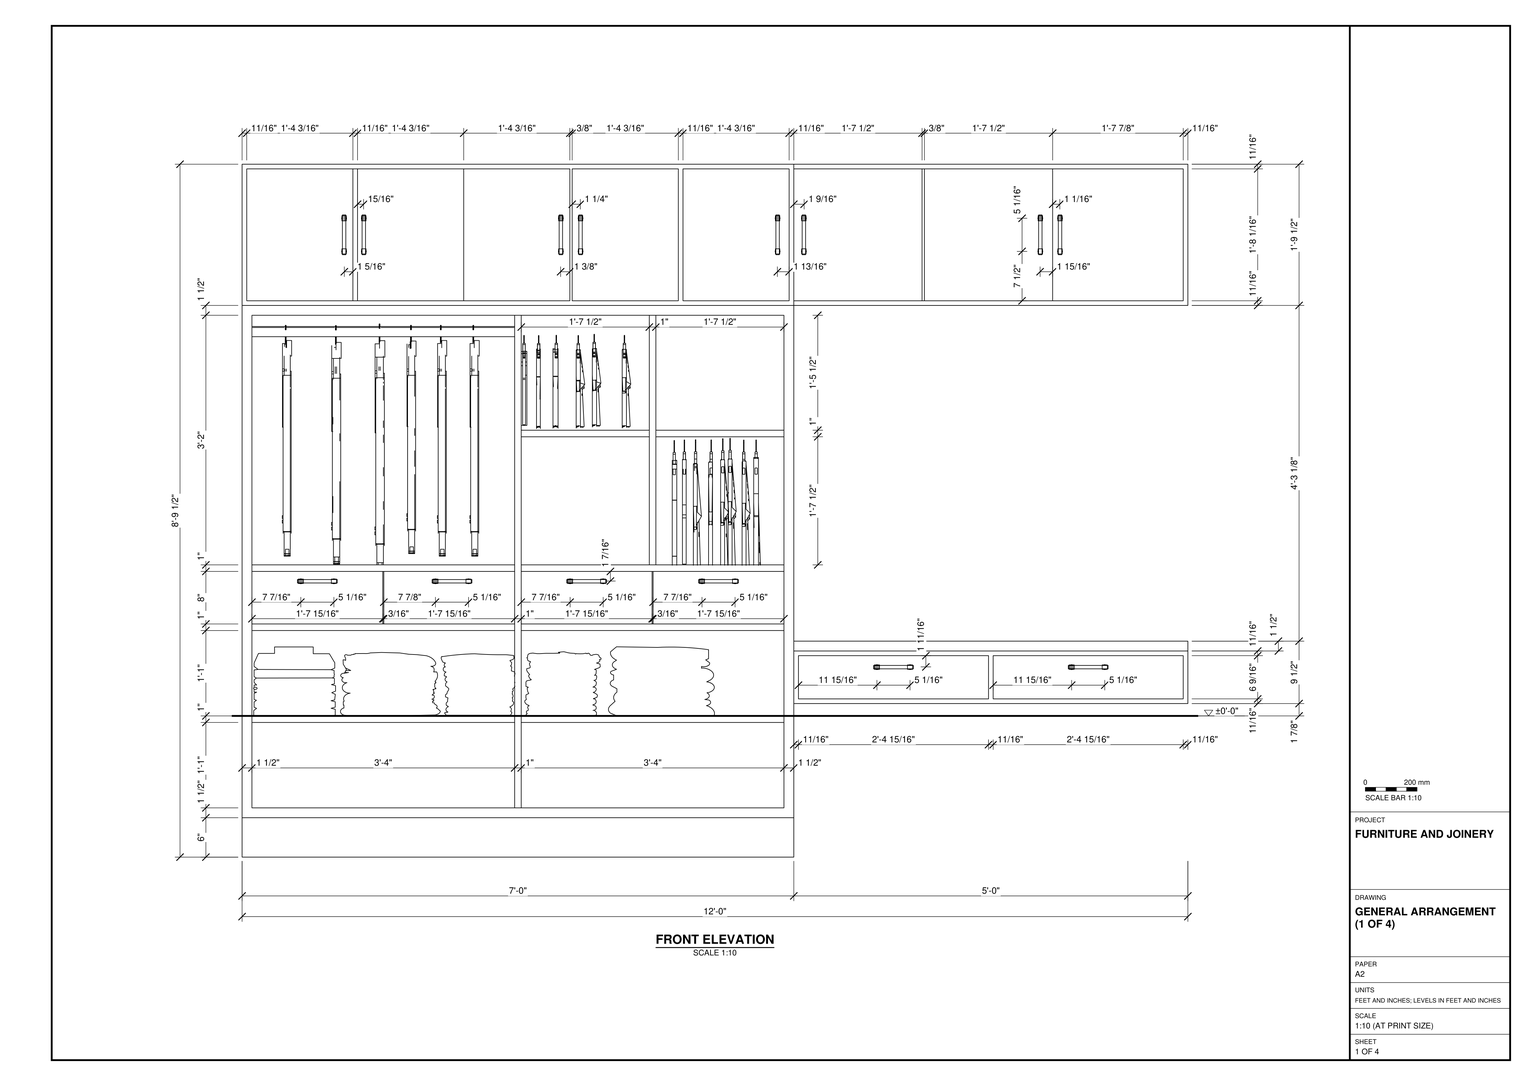
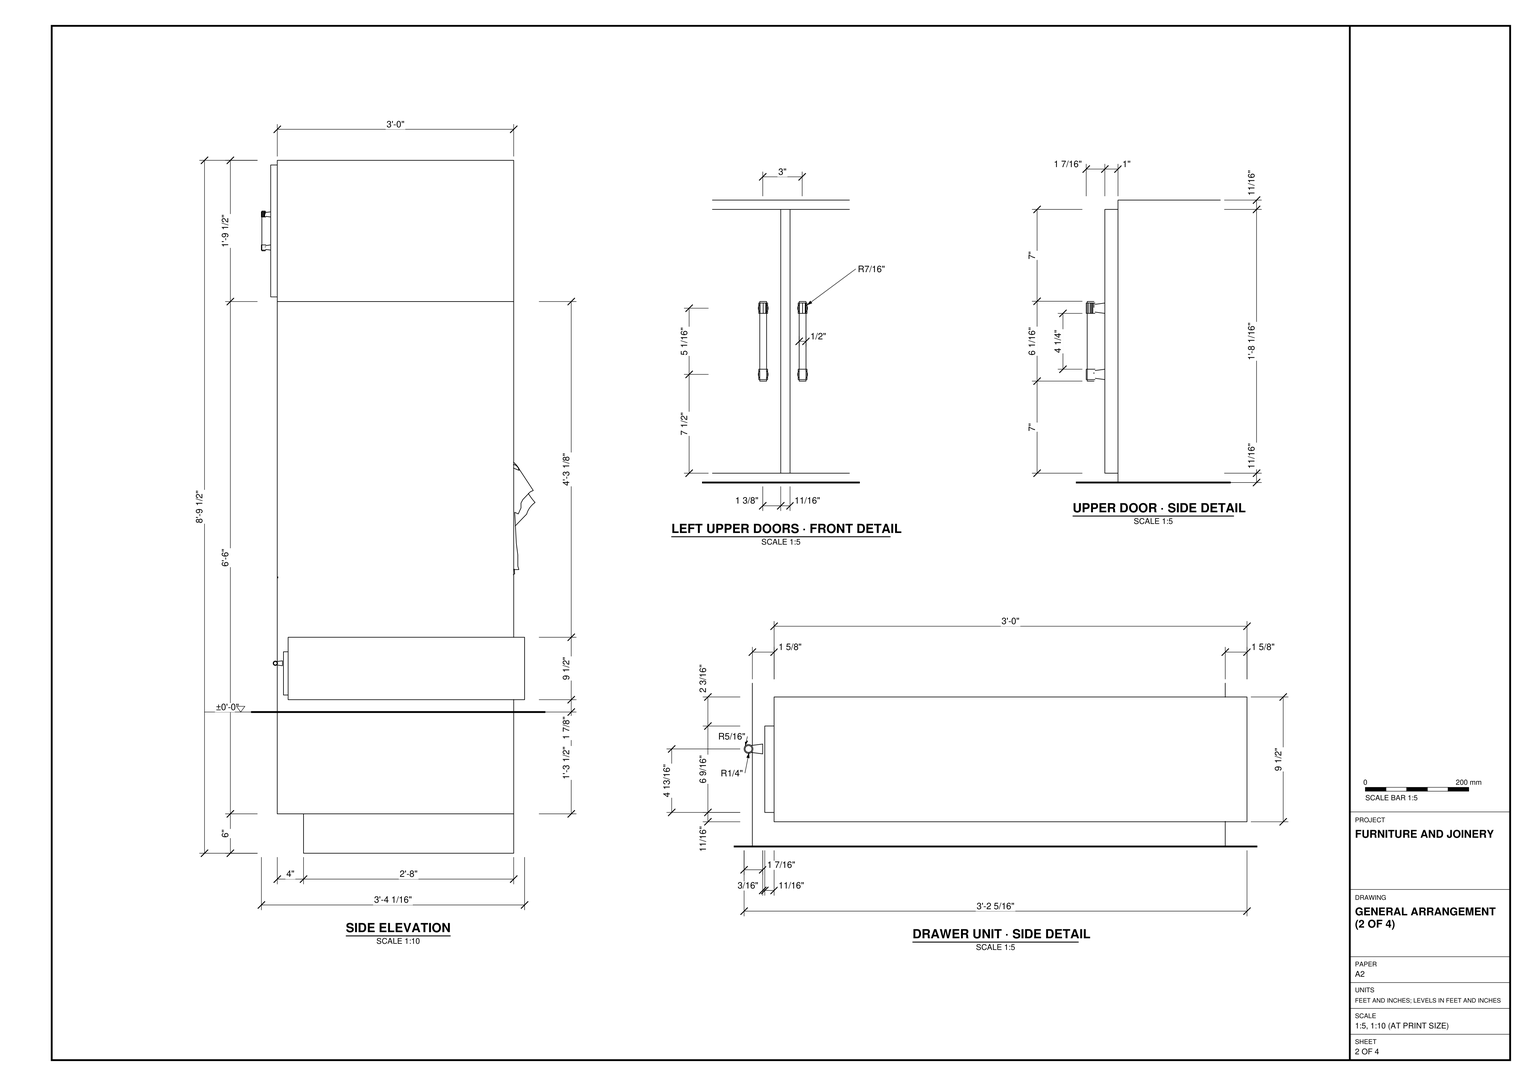
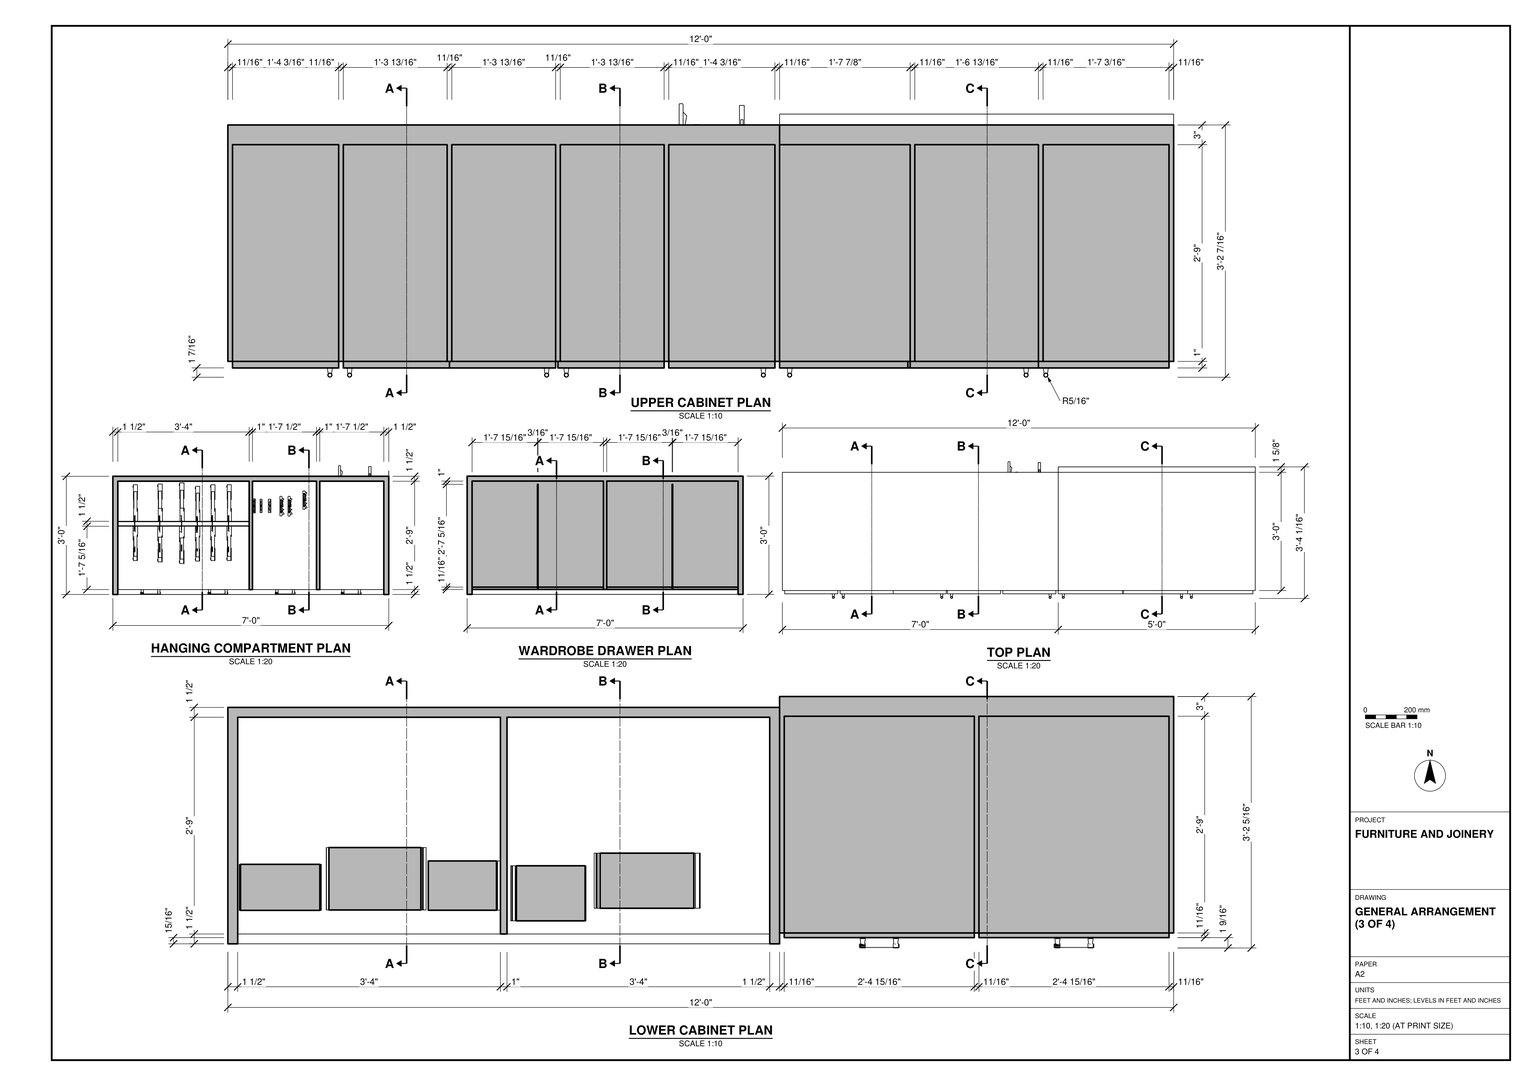
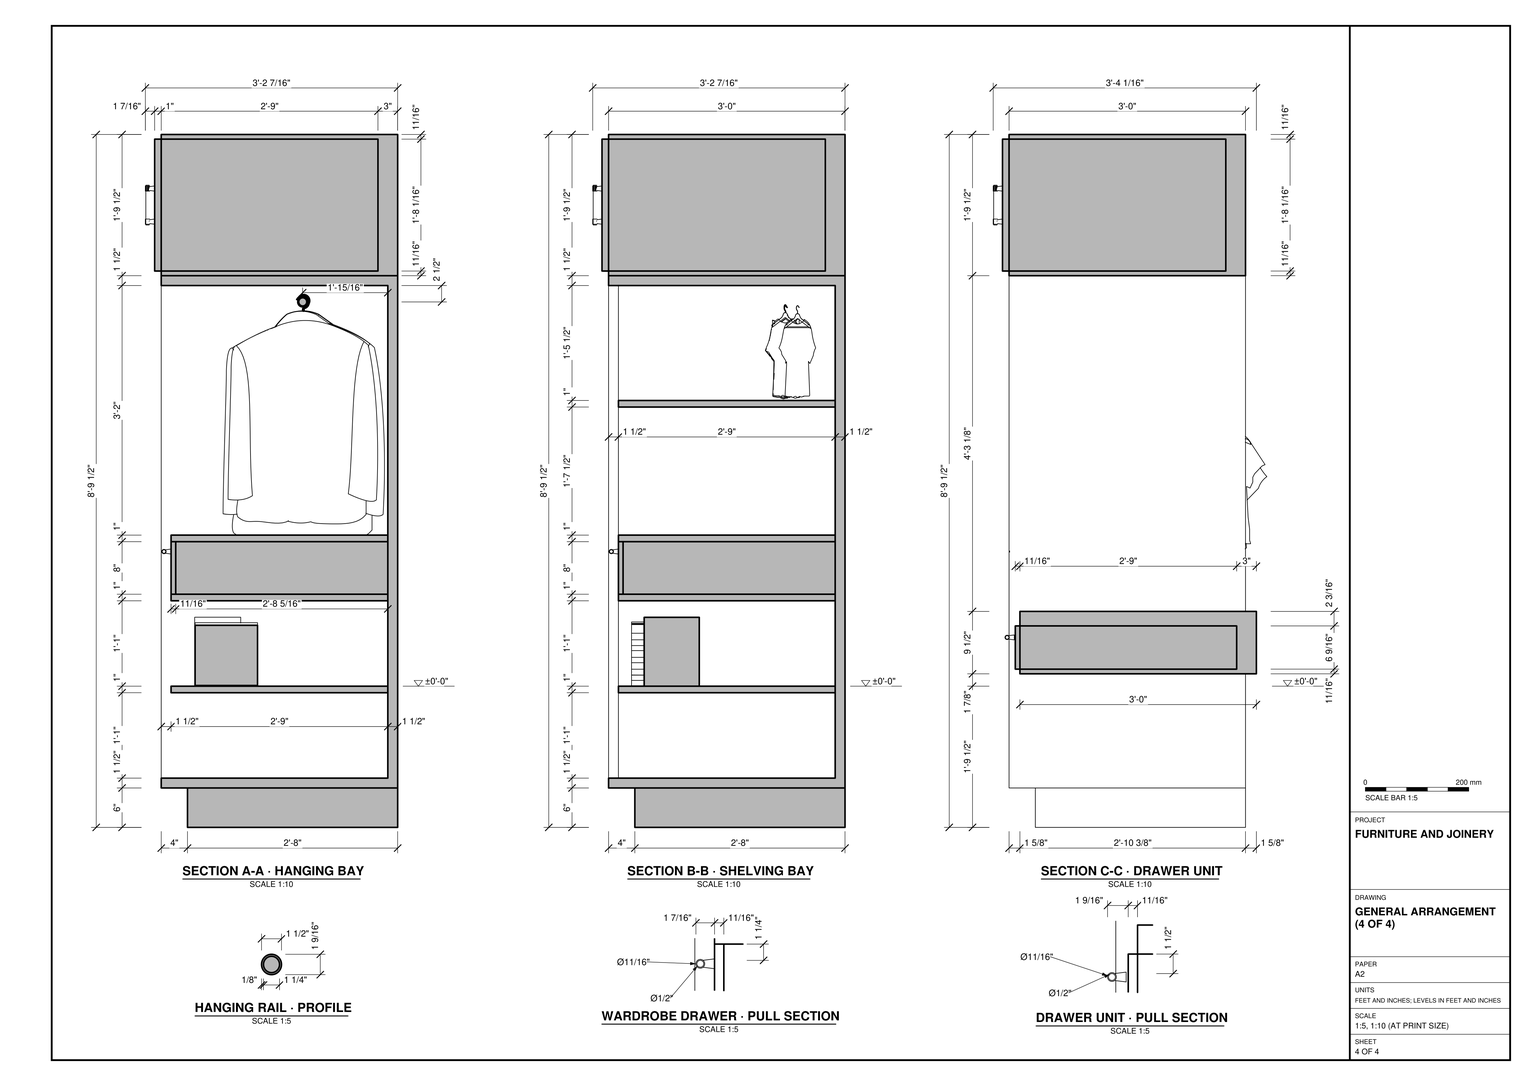
Build the wardrobe assembly in SketchUp from task_files/diagram_01.pdf. Work in feet and inches. The complete assembly is 12'-0" wide, 3'-5 11/16" deep and 8'-9 1/2" high. Use the ±0'-0" datum shown in the elevations; the wardrobe plinth sits below this line.

Set out the 7'-0" wardrobe on the left and the 5'-0" drawer unit on the right. Run the upper cabinets across both sections, following the door widths and pull positions in the front elevation. Below the left cabinets, form a wide bay for long garments and two narrower bays with intermediate shelves. Fit the row of drawers beneath the hanging bays, with divided open shelving and a recessed plinth below. On the right, leave the space between the suspended two-drawer unit and the overhead cabinets open. Use the plans and side details to set the panel thicknesses, front projections and pull orientations.

Place hanging garments and folded clothing in the compartments shown. Decor and loose items, including the clothing, may be any suitable library components. Keep each joinery piece in a separate group or component and use components for repeated parts such as matching pulls. Save one SketchUp model as output_files/wardrobe_with_overhead_cabinets_and_suspended_drawers.skp.

# SketchUp Ruby script. Lengths in inches.
U = 1.inch
M = Sketchup.active_model
def pt(a) = Geom::Point3d.new(a.map { |v| v * U })
def face(e, loops, mat)
  f = e.add_face(loops[0].map { |a| pt(a) })
  loops[1..].each { |l| e.add_face(l.map { |a| pt(a) }).erase! }
  f.material = f.back_material = mat if mat
  f
end
# faces: each face lists its corners as indices into pts; further lists are holes
def faces(e, pts, list, mat = nil) = list.each { |f| face(e, (f[0].is_a?(Array) ? f : [f]).map { |l| l.map { |i| pts[i] } }, mat) }
# xy, xz, yz: faces in a plane at the given z, y or x. An outline is a flat list of corners, or four numbers for a rectangle; further outlines are holes
def ring(l) = l.size == 4 ? [[l[0], l[1]], [l[2], l[1]], [l[2], l[3]], [l[0], l[3]]] : l.each_slice(2).to_a
def flat(e, list, mat, &to3) = list.each { |f| face(e, (f[0].is_a?(Array) ? f : [f]).map { |l| ring(l).map { |u, v| to3.(u, v) } }, mat) }
def xy(e, z, list, mat = nil) = flat(e, list, mat) { |x, y| [x, y, z] }
def xz(e, y, list, mat = nil) = flat(e, list, mat) { |x, z| [x, y, z] }
def yz(e, x, list, mat = nil) = flat(e, list, mat) { |y, z| [x, y, z] }
def lines(e, pts, list) = list.each { |a, b| e.add_line(pt(pts[a]), pt(pts[b])) }
# prism: a flat outline (further loops are holes) pulled along v
def prism(e, loops, v, mat = nil)
  f = face(e, loops, mat); d = Geom::Vector3d.new(v.map { |x| x * U })
  f.pushpull(f.normal.samedirection?(d) ? d.length : -d.length)
end
def box(e, o, s, mat = nil) = prism(e, [[o, [o[0] + s[0], o[1], o[2]], [o[0] + s[0], o[1] + s[1], o[2]], [o[0], o[1] + s[1], o[2]]]], [0, 0, s[2]], mat)
def at(x, y, z, deg = 0) = Geom::Transformation.translation(pt([x, y, z])) * Geom::Transformation.rotation(ORIGIN, Z_AXIS, deg.degrees)
def axes(o, x, y, z) = Geom::Transformation.new([*x, 0, *y, 0, *z, 0, *pt(o).to_a, 1])
def part(name) = M.definitions.add(name)
# library, detail: a bought-in or finely detailed component or shape, given as its bounding box
def library(name, o, s) = part(name).tap { |d| box(d.entities, o, s) }
def detail(e, o, s) = box(e.add_group.entities, o, s)
def put(e, d, t, mat = nil) = e.add_instance(d, t).tap { |i| i.material = mat if mat }
def group(e, t, mat = nil) = e.add_group.tap { |g| g.transformation = t; g.material = mat if mat }.entities
root = M.entities
c1 = library("1-POIGNEE CLC2",[-3.03,-0.375,0],[6.06,0.75,1.42])
c2 = library("clothing6",[65.37,-6.9,0.1],[26.12,44.83,39.07])
c3 = library("clothing (1)",[291.68,-309.73,41.26],[36.47,20.09,38.36])
c4 = library("Component",[186.95,333.1,21.5],[70.2,11.17,10.52])
c5 = part("Group\#3")
box(c5.entities,[0,0,0],[19.5,33,1])
c6 = part("Group\#7")
box(c6.entities,[0,0,0],[40,33,1])
c7 = part("Group\#14")
box(c7.entities,[0,0,0],[16.16,1,20.08])
c8 = part("Group\#13")
put(c8.entities,c7,at(0,-1,0))
c9 = part("Group\#16")
box(c9.entities,[0,-1,0],[19.88,1,20.08])
c10 = part("Group\#18")
box(c10.entities,[0,-0.71,0],[28.9375,0.71,6.58])
c11 = part("Group\#20")
box(c11.entities,[0,-0.71,0],[19.92,0.71,8])
prism(root,[[[1.5,35.5,35.5],[41.5,35.5,35.5],[41.5,3.21,35.5],[21.58,3.21,35.5],[21.58,34.5,35.5],[21.42,34.5,35.5],[21.42,3.21,35.5],[1.5,3.21,35.5]]],[0,0,8])
p = [[62,35.5,82.5],[62,35.5,44.5],[63,35.5,82.5],[63,35.5,44.5]]
lines(root,p,[[0,1],[2,3]])
put(root,c1,axes([11.46,2.5,42],[1,0,0],[0,0,1],[0,-1,0]))
put(root,c1,axes([31.96,2.5,42],[1,0,0],[0,0,1],[0,-1,0]))
put(root,c1,axes([52.46,2.5,42],[1,0,0],[0,0,1],[0,-1,0]))
put(root,c1,axes([72.54,2.5,42],[1,0,0],[0,0,1],[0,-1,0]))
put(root,c1,axes([99.18,1.79,28.93],[1,0,0],[0,0,1],[0,-1,0]))
put(root,c1,axes([15.53,0,94.75],[0,0,-1],[1,0,0],[0,-1,0]))
put(root,c1,axes([128.82,1.79,28.93],[1,0,0],[0,0,1],[0,-1,0]))
put(root,c1,axes([18.53,0,94.75],[0,0,-1],[1,0,0],[0,-1,0]))
put(root,c1,axes([48.53,0,94.75],[0,0,-1],[1,0,0],[0,-1,0]))
put(root,c1,axes([51.53,0,94.75],[0,0,-1],[1,0,0],[0,-1,0]))
put(root,c1,axes([81.53,0,94.75],[0,0,-1],[1,0,0],[0,-1,0]))
put(root,c1,axes([85.53,0,94.75],[0,0,-1],[1,0,0],[0,-1,0]))
put(root,c1,axes([121.53,0,94.75],[0,0,-1],[1,0,0],[0,-1,0]))
put(root,c1,axes([124.53,0,94.75],[0,0,-1],[1,0,0],[0,-1,0]))
put(root,c2,axes([7.66,96.49,43.61],[0,-0.9408,0],[0.89234,0,0],[0,0,0.95962]))
put(root,c3,at(-249.18,329.89,0))
put(root,c4,at(-185.22,-328.6,0))
put(root,c5,at(42.5,2.5,64))
g1 = group(root,at(42.5,2.5,43.5))
box(g1,[0,0,0],[40,33,1])
g2 = group(root,at(0,37,6))
xy(g2,0,[[0,-36,84,0]])
xy(g2,1.5,[[1.5,-36,82.5,-36,82.5,-1.5,42.5,-1.5,42.5,-34.5,41.5,-34.5,41.5,-1.5,1.5,-1.5]])
xy(g2,38.5,[[62,-34.5,63,-1.5]])
xy(g2,76.5,[[1.5,-36,1.5,-1.5,41.5,-1.5,41.5,-34.5,42.5,-34.5,42.5,-1.5,62,-1.5,62,-34.5,63,-34.5,63,-1.5,82.5,-1.5,82.5,-36]])
xy(g2,78,[[0,-36,84,0]])
xz(g2,-36,[[[0,0,84,78],[1.5,1.5,82.5,76.5]]])
xz(g2,-34.5,[[41.5,1.5,42.5,76.5],[62,38.5,63,76.5]])
xz(g2,-1.5,[[1.5,1.5,41.5,76.5],[42.5,1.5,82.5,1.5,82.5,76.5,63,76.5,63,38.5,62,38.5,62,76.5,42.5,76.5]])
xz(g2,0,[[0,0,84,78]])
yz(g2,0,[[-36,0,0,78]])
yz(g2,1.5,[[-36,1.5,-1.5,76.5]])
yz(g2,41.5,[[-34.5,1.5,-1.5,76.5]])
yz(g2,42.5,[[-34.5,1.5,-1.5,76.5]])
yz(g2,62,[[-34.5,38.5,-1.5,76.5]])
yz(g2,63,[[-34.5,38.5,-1.5,76.5]])
yz(g2,82.5,[[-36,1.5,-1.5,76.5]])
yz(g2,84,[[-36,0,0,78]])
put(root,c6,at(42.5,2.5,20.5))
g3 = group(root,at(42.5,2.5,34.5))
box(g3,[0,0,0],[40,33,1])
put(root,c6,at(1.5,2.5,20.5))
put(root,c6,at(1.5,2.5,34.5))
g4 = group(root,at(0,1,0))
box(g4,[0,4,0],[84,32,6])
put(root,c5,at(63,2.5,64))
g5 = group(root,at(42.5,35.5,35.5))
xy(g5,0,[[0,-32.29,0,0,40,0,40,-32.29,20.08,-32.29,20.08,-1,19.92,-1,19.92,-32.29]])
xy(g5,8,[[0,-32.29,19.92,-32.29,19.92,-1,20.08,-1,20.08,-32.29,40,-32.29,40,0,0,0]])
xz(g5,-32.29,[[0,0,19.92,8]])
xz(g5,-1,[[19.92,0,20.08,8]])
xz(g5,0,[[0,0,40,8]])
yz(g5,0,[[-32.29,0,0,8]])
yz(g5,19.92,[[-32.29,0,-1,8]])
yz(g5,20.08,[[-32.29,0,-1,8]])
yz(g5,40,[[-32.29,0,0,8]])
put(root,c6,at(1.5,2.5,43.5))
g6 = group(root,at(62.58,3.21,35.5))
xz(g6,0,[[0,0,19.92,8]])
g7 = group(root,at(1.5,35.5,35.5))
xz(g7,0,[[0,0,40,8]])
g8 = group(root,at(0,1,84))
xy(g8,0,[[0,0,84,36]])
xy(g8,0.71,[[0.71,0,16.87,33],[17.58,0,33.39,33],[34.1,0,49.9,33],[50.61,0,66.42,33],[67.13,0,83.29,33]])
xy(g8,20.79,[[0.71,0,16.87,33],[17.58,0,33.39,33],[34.1,0,49.9,33],[50.61,0,66.42,33],[67.13,0,83.29,33]])
xy(g8,21.5,[[0,0,84,36]])
xz(g8,0,[[[0,0,84,21.5],[0.71,0.71,33.39,20.79],[67.13,0.71,83.29,20.79],[50.61,0.71,66.42,20.79],[34.1,0.71,49.9,20.79]]])
xz(g8,33,[[0.71,0.71,16.87,20.79],[17.58,0.71,33.39,20.79],[34.1,0.71,49.9,20.79],[50.61,0.71,66.42,20.79],[67.13,0.71,83.29,20.79]])
xz(g8,36,[[0,0,84,21.5]])
yz(g8,0,[[0,0,36,21.5]])
yz(g8,0.71,[[0,0.71,33,20.79]])
yz(g8,16.87,[[0,0.71,33,20.79]])
yz(g8,17.58,[[0,0.71,33,20.79]])
yz(g8,33.39,[[0,0.71,33,20.79]])
yz(g8,34.1,[[0,0.71,33,20.79]])
yz(g8,49.9,[[0,0.71,33,20.79]])
yz(g8,50.61,[[0,0.71,33,20.79]])
yz(g8,66.42,[[0,0.71,33,20.79]])
yz(g8,67.13,[[0,0.71,33,20.79]])
yz(g8,83.29,[[0,0.71,33,20.79]])
yz(g8,84,[[0,0,36,21.5]])
g9 = group(g8,at(16.87,0,0.71))
xz(g9,0,[[0,0,0.71,20.08]])
g10 = group(root,at(84,1,84))
xy(g10,0,[[0,0,60,36]])
xy(g10,0.71,[[0,0,19.88,33],[20.59,0,39.41,33],[40.12,0,59.29,33]])
xy(g10,20.79,[[0,0,19.88,33],[20.59,0,39.41,33],[40.12,0,59.29,33]])
xy(g10,21.5,[[0,0,60,36]])
xz(g10,0,[[[0,0,60,0,60,21.5,0,21.5,0,20.79,19.88,20.79,19.88,0.71,0,0.71],[40.12,0.71,59.29,20.79],[20.59,0.71,39.41,20.79]]])
xz(g10,33,[[0,0.71,19.88,20.79],[20.59,0.71,39.41,20.79],[40.12,0.71,59.29,20.79]])
xz(g10,36,[[0,0,60,21.5]])
yz(g10,0,[[0,0,0,0.71,33,0.71,33,20.79,0,20.79,0,21.5,36,21.5,36,0]])
yz(g10,19.88,[[0,0.71,33,20.79]])
yz(g10,20.59,[[0,0.71,33,20.79]])
yz(g10,39.41,[[0,0.71,33,20.79]])
yz(g10,40.12,[[0,0.71,33,20.79]])
yz(g10,59.29,[[0,0.71,33,20.79]])
yz(g10,60,[[0,0,36,21.5]])
put(root,c8,at(17.58,1,84.71))
put(root,c8,at(67.13,1,84.71))
put(root,c8,at(50.26,1,84.71))
put(root,c8,at(33.74,1,84.71))
g11 = group(root,at(0.71,1,84.71))
put(g11,c7,at(0,-1,0))
put(root,c9,at(84,1,84.71))
put(root,c9,at(103.53,1,84.71))
put(root,c9,at(123.41,1,84.71))
g12 = group(root,at(84,2.66,23.38))
xy(g12,0,[[0,0,60,36]])
xy(g12,0.71,[[0.71,0,29.65,33],[30.35,0,59.29,33]])
xy(g12,7.29,[[0.71,0,29.65,33],[30.35,0,59.29,33]])
xy(g12,9.5,[[0,0,60,36]])
xz(g12,0,[[[0,0,60,8],[0.71,0.71,29.65,7.29],[30.35,0.71,59.29,7.29]],[0,8,60,9.5]])
xz(g12,33,[[0.71,0.71,29.65,7.29],[30.35,0.71,59.29,7.29]])
xz(g12,36,[[0,0,60,9.5]])
yz(g12,0,[[0,0,36,9.5]])
yz(g12,0.71,[[0,0.71,33,7.29]])
yz(g12,29.65,[[0,0.71,33,7.29]])
yz(g12,30.35,[[0,0.71,33,7.29]])
yz(g12,59.29,[[0,0.71,33,7.29]])
yz(g12,60,[[0,0,36,9.5]])
put(root,c10,at(84.71,2.66,24.09))
put(root,c10,at(114.35,2.66,24.09))
put(root,c11,at(42.5,3.21,35.5))
put(root,c11,at(62.58,3.21,35.5))
put(root,c11,at(1.5,3.21,35.5))
g13 = group(root,at(21.58,3.21,35.5))
box(g13,[0,-0.71,0],[19.92,0.71,8])
